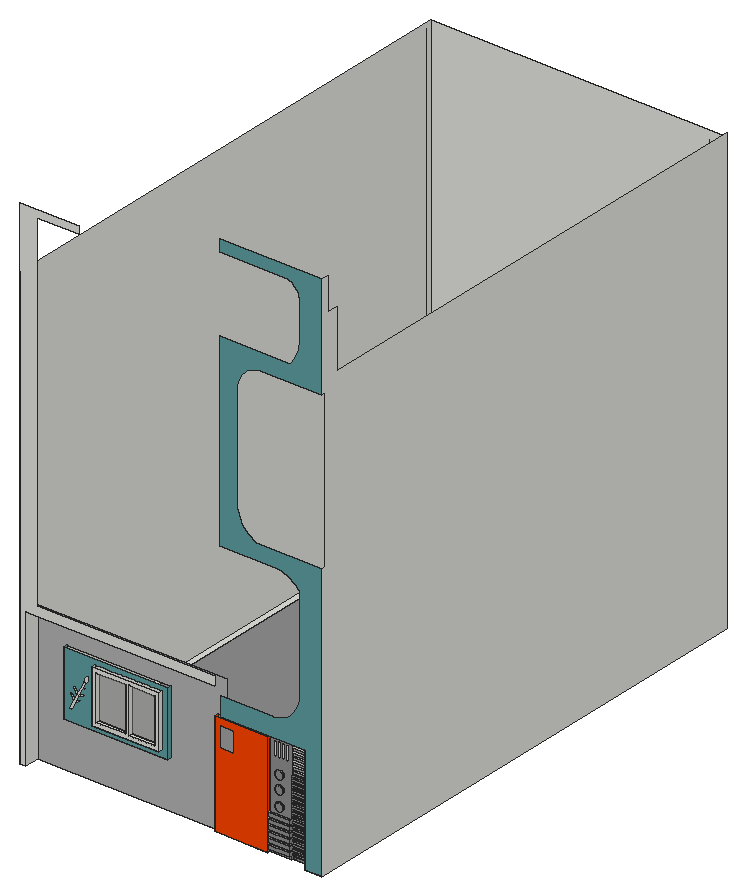
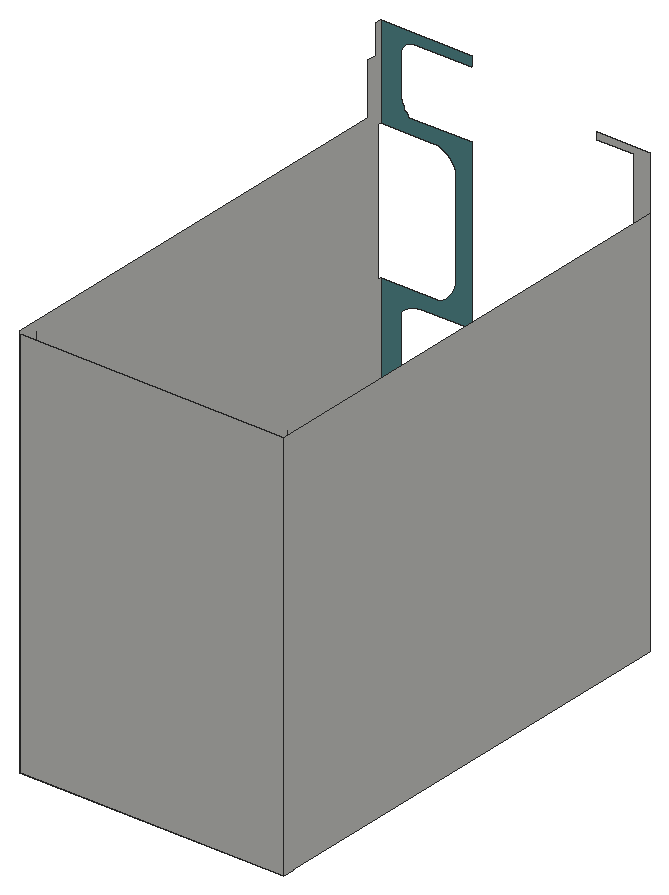
# SketchUp Ruby script. Lengths in inches.
U = 1.inch
M = Sketchup.active_model
def pt(a) = Geom::Point3d.new(a.map { |v| v * U })
def face(e, loops, mat)
  f = e.add_face(loops[0].map { |a| pt(a) })
  loops[1..].each { |l| e.add_face(l.map { |a| pt(a) }).erase! }
  f.material = f.back_material = mat if mat
  f
end
# faces: each face lists its corners as indices into pts; further lists are holes
def faces(e, pts, list, mat = nil) = list.each { |f| face(e, (f[0].is_a?(Array) ? f : [f]).map { |l| l.map { |i| pts[i] } }, mat) }
# xy, xz, yz: faces in a plane at the given z, y or x. An outline is a flat list of corners, or four numbers for a rectangle; further outlines are holes
def ring(l) = l.size == 4 ? [[l[0], l[1]], [l[2], l[1]], [l[2], l[3]], [l[0], l[3]]] : l.each_slice(2).to_a
def flat(e, list, mat, &to3) = list.each { |f| face(e, (f[0].is_a?(Array) ? f : [f]).map { |l| ring(l).map { |u, v| to3.(u, v) } }, mat) }
def xy(e, z, list, mat = nil) = flat(e, list, mat) { |x, y| [x, y, z] }
def xz(e, y, list, mat = nil) = flat(e, list, mat) { |x, z| [x, y, z] }
def yz(e, x, list, mat = nil) = flat(e, list, mat) { |y, z| [x, y, z] }
def lines(e, pts, list) = list.each { |a, b| e.add_line(pt(pts[a]), pt(pts[b])) }
# prism: a flat outline (further loops are holes) pulled along v
def prism(e, loops, v, mat = nil)
  f = face(e, loops, mat); d = Geom::Vector3d.new(v.map { |x| x * U })
  f.pushpull(f.normal.samedirection?(d) ? d.length : -d.length)
end
def box(e, o, s, mat = nil) = prism(e, [[o, [o[0] + s[0], o[1], o[2]], [o[0] + s[0], o[1] + s[1], o[2]], [o[0], o[1] + s[1], o[2]]]], [0, 0, s[2]], mat)
def at(x, y, z, deg = 0) = Geom::Transformation.translation(pt([x, y, z])) * Geom::Transformation.rotation(ORIGIN, Z_AXIS, deg.degrees)
def axes(o, x, y, z) = Geom::Transformation.new([*x, 0, *y, 0, *z, 0, *pt(o).to_a, 1])
def part(name) = M.definitions.add(name)
# library, detail: a bought-in or finely detailed component or shape, given as its bounding box
def library(name, o, s) = part(name).tap { |d| box(d.entities, o, s) }
def detail(e, o, s) = box(e.add_group.entities, o, s)
def put(e, d, t, mat = nil) = e.add_instance(d, t).tap { |i| i.material = mat if mat }
def group(e, t, mat = nil) = e.add_group.tap { |g| g.transformation = t; g.material = mat if mat }.entities
root = M.entities
M.materials.add("Niraj_Hair_Gray").color = [178, 178, 178]
M.materials.add("[0024_OrangeRed]").color = [255, 69, 0]
M.materials.add("[0081_CadetBlue]").color = [95, 158, 160]
M.materials.add("[Color M04]").color = [142, 142, 142]
M.materials.add("[Translucent Glass Gray]").color = [128, 128, 128]
M.materials["[Translucent Glass Gray]"].alpha = 0.5
xy(root,-2,[[198.26,11,216.37,12]])
xy(root,-2,[[230.7,6,230.7,12,198.26,12,198.26,9,153.86,9,153.86,12,5,12,5,414.4375,0,414.4375,0,424.625,245.1875,424.625,245.1875,6]],"[Color M04]")
xy(root,-1.875,[[0,0,5,414.4375]])
xy(root,0.7,[[198.26,9,216.37,11]],"[Color M04]")
xy(root,1.375,[[216.37,11,230.7,12]])
xy(root,2.67,[[216.37,11,230.7,12]],"[Color M04]")
xy(root,3.79,[[198.26,9,216.37,11]],"[Color M04]")
xy(root,4.8125,[[216.37,11,230.7,12]])
xy(root,5.51,[[198.26,9,216.37,11]])
xy(root,6.1,[[216.37,11,230.7,12]])
xy(root,8.25,[[216.37,11,230.7,12]])
xy(root,8.6,[[198.26,9,216.37,11]],"[Color M04]")
xy(root,9.54,[[216.37,11,230.7,12]])
xy(root,10.32,[[198.26,9,216.37,11]])
xy(root,11.6875,[[216.37,11,230.7,12]])
xy(root,12.98,[[216.37,11,230.7,12]])
xy(root,13.42,[[198.26,9,216.37,11]],"[Color M04]")
xy(root,15.125,[[216.37,11,230.7,12]])
xy(root,15.14,[[198.26,9,216.37,11]])
xy(root,16.42,[[216.37,11,230.7,12]])
xy(root,18.23,[[198.26,9,216.37,11]],"[Color M04]")
xy(root,18.5625,[[216.37,11,230.7,12]])
xy(root,19.85,[[216.37,11,230.7,12]])
xy(root,19.95,[[198.26,9,216.37,11]])
xy(root,22,[[216.37,11,230.7,12]])
xy(root,23.04,[[198.26,9,216.37,11]],"[Color M04]")
xy(root,23.29,[[216.37,11,230.7,12]])
xy(root,24.76,[[198.26,9,216.37,11]])
xy(root,25.4375,[[216.37,11,230.7,12]])
xy(root,26.73,[[216.37,11,230.7,12]])
xy(root,27.85,[[198.26,9,216.37,11]],"[Color M04]")
xy(root,28.875,[[216.37,11,230.7,12]])
xy(root,30.17,[[216.37,11,230.7,12]])
xy(root,32.3125,[[216.37,11,230.7,12]])
xy(root,33.6,[[216.37,11,230.7,12]])
xy(root,35.75,[[216.37,11,230.7,12]])
xy(root,37.04,[[216.37,11,230.7,12]])
xy(root,37.67,[[29.19,9,114.82,12]],"[0081_CadetBlue]")
xy(root,39.1875,[[216.37,11,230.7,12]])
xy(root,40.48,[[216.37,11,230.7,12]])
xy(root,42.625,[[216.37,11,230.7,12]])
xy(root,43.17,[[54.96,6,110.28,9]])
xy(root,43.92,[[216.37,11,230.7,12]])
xy(root,46.0625,[[216.37,11,230.7,12]])
xy(root,46.33,[[58.13,6,82.62,9],[85.26,6,107.11,9]])
xy(root,47.35,[[216.37,11,230.7,12]])
xy(root,49.5,[[216.37,11,230.7,12]])
xy(root,50.79,[[216.37,11,230.7,12]])
xy(root,52.9375,[[216.37,11,230.7,12]])
xy(root,54.23,[[216.37,11,230.7,12]])
xy(root,56.375,[[216.37,11,230.7,12]])
xy(root,57.67,[[216.37,11,230.7,12]])
xy(root,59.8125,[[216.37,11,230.7,12]])
xz(root,0,[[0,-1.875,5,-1.875,5,112.3125,161.25,112.3125,161.25,120,14,120,14,407.79,48.4375,407.79,48.4375,414,0,414]])
xz(root,6,[[[54.96,43.17,110.28,86.73],[58.13,46.33,82.62,83.5625],[85.26,46.33,107.11,83.5625]]])
xz(root,6,[[230.7,-2,245.1875,-2,245.1875,226.28,190.26,226.28,188.03,227.37,185.92,228.66,183.95,230.16,182.125,231.84,180.47,233.68,179.01,235.68,177.75,237.82,176.7,240.0625,175.87,242.4,175.28,244.8,174.92,247.25,174.8,249.73,174.8,334.1,174.98,336.86,175.52,339.57,176.41,342.19,177.63,344.68,179.17,346.98,180.99,349.06,183.07,350.88,185.375,352.42,187.86,353.65,190.48,354.54,193.19,355.08,195.95,355.26,245.1875,355.26,245.1875,441.0625,160.53,441.0625,160.53,431.57,212.95,431.57,214.73,431.46,216.48,431.11,218.17,430.54,219.77,429.75,221.25,428.76,222.6,427.58,223.77,426.24,224.76,424.76,225.55,423.16,226.125,421.47,226.47,419.72,226.59,417.9375,226.59,388.52,226.53,386.72,226.36,384.93,226.08,383.15,225.6875,381.39,225.1875,379.66,224.57,377.97,223.86,376.32,223.04,374.72,222.125,373.17,221.11,371.68,220.01,370.26,218.8125,368.91,160.53,368.91,160.53,213.14,206.79,213.14,208.72,213.07,210.64,212.84,212.53,212.45,214.39,211.92,216.19,211.24,217.94,210.42,219.62,209.47,221.22,208.38,222.72,207.17,224.12,205.84,225.42,204.41,226.59,202.88,226.59,125.26,226.39,122.24,225.8,119.26,224.82,116.39,223.48,113.66,221.8,111.14,219.8,108.86,217.51,106.86,214.99,105.17,212.27,103.83,209.4,102.86,206.42,102.26,203.39,102.07,161.25,102.07,161.25,86.5625,230.7,86.5625]],"[0081_CadetBlue]")
xz(root,9,[[[54.96,43.17,110.28,86.73],[58.13,46.33,82.62,83.5625],[85.26,46.33,107.11,83.5625]],[33.9375,47.49,35.62,47.49,38.55,53.26,41.47,59.04,44.14,64.29,46.5,68.96,47.17,70.28,46.5,70.62,45.84,70.96,45.41,70.12,42.7,64.77,40.01,59.47,36.97,53.48],[38.55,53.26,44.04,55.68,43.51,55.74,42.99,55.74,42.46,55.7,41.94,55.61,41.43,55.46,40.9375,55.27,40.47,55.04,40.02,54.76,39.6,54.4375,39.21,54.08,38.86,53.6875],[36.97,53.48,37.22,53.99,37.375,54.53,37.45,55.09,37.43,55.65,37.33,56.2,37.14,56.73,36.87,57.23,36.53,57.67,36.12,58.0625,35.65,58.38,35.15,58.625,34.61,58.78],[41.47,59.04,46.18,60.52,45.76,60.62,45.33,60.68,44.89,60.7,44.46,60.67,44.03,60.6,43.6,60.49,43.2,60.34,42.8,60.15,42.43,59.92,42.08,59.66,41.76,59.36],
  [40.01,59.47,40.1875,59.97,40.29,60.48,40.31,61.01,40.25,61.54,40.12,62.05,39.92,62.54,39.64,62.99,39.3,63.4,38.91,63.75,38.47,64.04,37.99,64.27,37.48,64.42]])
xz(root,9,[[[153.86,-2,198.26,83.875],[157.99,61.11,169.99,78.23]]],"[0024_OrangeRed]")
xz(root,9,[[[29.19,37.67,114.82,90.99],[54.96,43.17,110.28,86.73],[33.9375,47.49,36.97,53.48,36.47,53.68,35.99,53.95,35.56,54.28,35.17,54.67,34.85,55.11,34.59,55.6,34.4,56.11,34.29,56.65,34.26,57.19,34.3,57.74,34.41,58.27,34.61,58.78,35.15,58.625,35.65,58.38,36.12,58.0625,36.53,57.67,36.87,57.23,37.14,56.73,37.33,56.2,37.43,55.65,37.45,55.09,37.375,54.53,37.22,53.99,36.97,53.48,34.61,58.78,34.41,58.27,34.3,57.74,34.26,57.19,34.29,56.65,34.4,56.11,34.59,55.6,34.85,55.11,35.17,54.67,35.56,54.28,35.99,53.95,36.47,53.68,36.97,53.48,40.01,59.47,39.5625,59.69,39.14,59.97,38.76,60.29,38.41,60.65,38.11,61.06,37.86,61.49,37.65,61.95,37.51,62.43,37.41,62.92,37.38,63.42,37.4,63.92,37.48,64.42,37.99,64.27,38.47,64.04,38.91,63.75,39.3,63.4,39.64,62.99,39.92,62.54,40.12,62.05,40.25,61.54,40.31,61.01,40.29,60.48,40.1875,59.97,40.01,59.47,37.48,64.42,37.4,63.92,37.38,63.42,37.41,62.92,37.51,62.43,37.65,61.95,37.86,61.49,38.11,61.06,38.41,60.65,38.76,60.29,39.14,59.97,39.5625,59.69,40.01,59.47,42.7,64.77,42.22,65.04,41.78,65.38,41.4,65.78,41.08,66.23,40.82,66.72,40.65,67.25,40.55,67.79,40.53,68.34,40.6,68.89,40.74,69.43,40.96,69.93,41.26,70.4,41.69,70.09,42.08,69.73,42.42,69.32,42.71,68.87,42.9375,68.38,43.1,67.875,43.2,67.35,43.23,66.82,43.2,66.29,43.1,65.76,42.93,65.26,42.7,64.77,41.26,70.4,40.96,69.93,40.74,69.43,40.6,68.89,40.53,68.34,40.55,67.79,40.65,67.25,40.82,66.72,41.08,66.23,41.4,65.78,41.78,65.38,42.22,65.04,42.7,64.77,45.41,70.12,45.28,70.83,45.25,71.5625,45.33,72.29,45.5,73,45.78,73.67,46.14,74.3,46.6,74.875,47.125,75.38,47.72,75.8,48.37,76.14,49.06,76.38,49.77,76.52,49.9,75.8,49.94,75.07,49.91,74.33,49.81,73.61,49.625,72.9,49.37,72.21,49.04,71.55,48.65,70.93,48.19,70.36,47.68,69.83,47.12,69.36,46.5,68.96,44.14,64.29,44.64,64.2,45.14,64.17,45.65,64.1875,46.15,64.27,46.64,64.41,47.11,64.6,47.55,64.85,47.96,65.14,48.34,65.48,48.68,65.86,48.97,66.27,49.21,66.72,44.14,64.29,44.39,64.73,44.6875,65.13,45.03,65.5,45.41,65.83,45.82,66.12,46.26,66.36,46.73,66.55,47.21,66.7,47.71,66.78,48.21,66.81,48.72,66.79,49.21,66.72,48.97,66.27,48.68,65.86,48.34,65.48,47.96,65.14,47.55,64.85,47.11,64.6,46.64,64.41,46.15,64.27,45.65,64.1875,45.14,64.17,44.64,64.2,44.14,64.29,41.47,59.04,41.9,58.9,42.33,58.8,42.77,58.76,43.22,58.77,43.66,58.83,44.09,58.94,44.51,59.1,44.9,59.3,45.27,59.55,45.61,59.84,45.92,60.16,46.18,60.52,41.47,59.04,41.76,59.36,42.08,59.66,42.43,59.92,42.8,60.15,43.2,60.34,43.6,60.49,44.03,60.6,44.46,60.67,44.89,60.7,45.33,60.68,45.76,60.62,46.18,60.52,45.92,60.16,45.61,59.84,45.27,59.55,44.9,59.3,44.51,59.1,44.09,58.94,43.66,58.83,43.22,58.77,42.77,58.76,42.33,58.8,41.9,58.9,41.47,59.04,38.55,53.26,39.08,53.17,39.61,53.13,40.15,53.15,40.68,53.23,41.19,53.37,41.7,53.56,42.17,53.8,42.625,54.09,43.04,54.43,43.42,54.81,43.75,55.23,44.04,55.68,38.55,53.26,38.86,53.6875,39.21,54.08,39.6,54.4375,40.02,54.76,40.47,55.04,40.9375,55.27,41.43,55.46,41.94,55.61,42.46,55.7,42.99,55.74,43.51,55.74,44.04,55.68,43.75,55.23,43.42,54.81,43.04,54.43,42.625,54.09,42.17,53.8,41.7,53.56,41.19,53.37,40.68,53.23,40.15,53.15,39.61,53.13,39.08,53.17,38.55,53.26,35.62,47.49]]],"[0081_CadetBlue]")
xz(root,9,[[198.26,0.7,216.37,3.79],[198.26,5.51,216.37,8.6],[198.26,10.32,216.37,13.42],[198.26,15.14,216.37,18.23],[198.26,19.95,216.37,23.04],
  [198.26,24.76,216.37,27.85]],"[Color M04]")
xz(root,9,[[58.13,46.33,82.62,83.5625],[85.26,46.33,107.11,83.5625]],"[Translucent Glass Gray]")
xz(root,10,[[206.34,30.52,207.21,30.63,208.03,30.97,208.73,31.5,209.26,32.2,209.6,33.02,209.71,33.89,209.6,34.76,209.26,35.58,208.73,36.28,208.03,36.8125,207.21,37.15,206.34,37.27,205.47,37.15,204.65,36.8125,203.95,36.28,203.42,35.58,203.08,34.76,202.96,33.89,203.08,33.02,203.42,32.2,203.95,31.5,204.65,30.97,205.47,30.63],[206.34,43.2,207.21,43.32,208.03,43.66,208.73,44.19,209.26,44.89,209.6,45.7,209.71,46.58,209.6,47.45,209.26,48.27,208.73,48.96,208.03,49.5,207.21,49.84,206.34,49.95,205.47,49.84,204.65,49.5,203.95,48.96,203.42,48.27,203.08,47.45,202.96,46.58,203.08,45.7,203.42,44.89,203.95,44.19,204.65,43.66,205.47,43.32],[206.34,54.39,207.21,54.51,208.03,54.84,208.73,55.38,209.26,56.08,209.6,56.89,209.71,57.77,209.6,58.64,209.26,59.45,208.73,60.15,208.03,60.6875,207.21,61.03,206.34,61.14,205.47,61.03,204.65,60.6875,203.95,60.15,203.42,59.45,203.08,58.64,202.96,57.77,203.08,56.89,203.42,56.08,203.95,55.38,204.65,54.84,205.47,54.51]],"[Color M04]")
xz(root,11,[[198.26,-2,216.37,0.7],[216.37,1.375,230.7,2.67],[198.26,3.79,216.37,5.51],[216.37,4.8125,230.7,6.1],[216.37,8.25,230.7,9.54],
  [198.26,8.6,216.37,10.32],[216.37,11.6875,230.7,12.98],[198.26,13.42,216.37,15.14],[216.37,15.125,230.7,16.42],[198.26,18.23,216.37,19.95],
  [216.37,18.5625,230.7,19.85],[216.37,22,230.7,23.29],[198.26,23.04,216.37,24.76],[216.37,25.4375,230.7,26.73],[[198.26,27.85,216.37,83.875],[206.34,30.52,205.47,30.63,204.65,30.97,203.95,31.5,203.42,32.2,203.08,33.02,202.96,33.89,203.08,34.76,203.42,35.58,203.95,36.28,204.65,36.8125,205.47,37.15,206.34,37.27,207.21,37.15,208.03,36.8125,208.73,36.28,209.26,35.58,209.6,34.76,209.71,33.89,209.6,33.02,209.26,32.2,208.73,31.5,208.03,30.97,207.21,30.63],[206.34,43.2,205.47,43.32,204.65,43.66,203.95,44.19,203.42,44.89,203.08,45.7,202.96,46.58,203.08,47.45,203.42,48.27,203.95,48.96,204.65,49.5,205.47,49.84,206.34,49.95,207.21,49.84,208.03,49.5,208.73,48.96,209.26,48.27,209.6,47.45,209.71,46.58,209.6,45.7,209.26,44.89,208.73,44.19,208.03,43.66,207.21,43.32],[206.34,54.39,205.47,54.51,204.65,54.84,203.95,55.38,203.42,56.08,203.08,56.89,202.96,57.77,203.08,58.64,203.42,59.45,203.95,60.15,204.65,60.6875,205.47,61.03,206.34,61.14,207.21,61.03,208.03,60.6875,208.73,60.15,209.26,59.45,209.6,58.64,209.71,57.77,209.6,56.89,209.26,56.08,208.73,55.38,208.03,54.84,207.21,54.51],[211.55,69.76,213.55,81.89],[208.18,69.76,210.18,81.89],[204.8,69.76,206.8,81.89],[201.43,69.76,203.43,81.89]],
  [216.37,28.875,230.7,30.17],[216.37,32.3125,230.7,33.6],[216.37,35.75,230.7,37.04],[216.37,39.1875,230.7,40.48],[216.37,42.625,230.7,43.92],
  [216.37,46.0625,230.7,47.35],[216.37,49.5,230.7,50.79],[216.37,52.9375,230.7,54.23],[216.37,56.375,230.7,57.67],[216.37,59.8125,230.7,61.1]],"[Color M04]")
xz(root,12,[[198.26,-2,216.37,-1.9375],[216.37,-2,230.7,-1.9375],[198.26,-1.9375,216.37,-1.875],[198.26,-1.875,216.37,0],[198.26,0,198.26,83.875,216.37,83.875,216.37,81.73,230.7,81.73,230.7,80.4375,216.37,80.4375,216.37,78.29,230.7,78.29,230.7,77,216.37,77,216.37,74.85,230.7,74.85,230.7,73.5625,216.37,73.5625,216.37,71.42,230.7,71.42,230.7,70.125,216.37,70.125,216.37,67.98,230.7,67.98,230.7,66.6875,216.37,66.6875,216.37,64.54,230.7,64.54,230.7,63.25,216.37,63.25,216.37,61.1,230.7,61.1,230.7,59.8125,216.37,59.8125,216.37,57.67,230.7,57.67,230.7,56.375,216.37,56.375,216.37,54.23,230.7,54.23,230.7,52.9375,216.37,52.9375,216.37,50.79,230.7,50.79,230.7,49.5,216.37,49.5,216.37,47.35,230.7,47.35,230.7,46.0625,216.37,46.0625,216.37,43.92,230.7,43.92,230.7,42.625,216.37,42.625,216.37,40.48,230.7,40.48,230.7,39.1875,216.37,39.1875,216.37,37.04,230.7,37.04,230.7,35.75,216.37,35.75,216.37,33.6,230.7,33.6,230.7,32.3125,216.37,32.3125,216.37,30.17,230.7,30.17,230.7,28.875,216.37,28.875,216.37,26.73,230.7,26.73,230.7,25.4375,216.37,25.4375,216.37,23.29,230.7,23.29,230.7,22,216.37,22,216.37,19.85,230.7,19.85,230.7,18.5625,216.37,18.5625,216.37,16.42,230.7,16.42,230.7,15.125,216.37,15.125,216.37,12.98,230.7,12.98,230.7,11.6875,216.37,11.6875,216.37,9.54,230.7,9.54,230.7,8.25,216.37,8.25,216.37,6.1,230.7,6.1,230.7,4.8125,216.37,4.8125,216.37,2.67,230.7,2.67,230.7,1.375,216.37,1.375,216.37,0],
  [29.19,37.67,114.82,81.74]])
xz(root,12,[[[5,-2,153.86,-2,153.86,83.875,230.7,83.875,230.7,86.5625,161.25,86.5625,161.25,112.3125,5,112.3125],[29.19,37.67,114.82,90.99]]],"Niraj_Hair_Gray")
xz(root,12,[[216.37,-1.9375,230.7,0]],"[Color M04]")
xz(root,414.4375,[[0,-2,5,-1.9375],[0,-1.9375,5,-1.875]])
xz(root,424.625,[[0,-2,245.1875,363]])
yz(root,0,[[414.4375,-2,414.4375,-1.875,0,-1.875,0,363,424.625,363,424.625,-2]])
yz(root,5,[[12,-2,414.4375,-1.9375],[12,-1.9375,414.4375,-1.875],[0,-1.875,12,112.3125]])
yz(root,29.19,[[9,37.67,12,90.99]],"[0081_CadetBlue]")
yz(root,54.96,[[6,43.17,9,86.73]])
yz(root,58.13,[[6,46.33,9,83.5625]])
yz(root,82.62,[[6,46.33,9,83.5625]])
yz(root,85.26,[[6,46.33,9,83.5625]])
yz(root,107.11,[[6,46.33,9,83.5625]])
yz(root,110.28,[[6,43.17,9,86.73]])
yz(root,114.82,[[9,37.67,12,90.99]],"[0081_CadetBlue]")
yz(root,153.86,[[9,-2,12,83.875]],"[0024_OrangeRed]")
yz(root,198.26,[[9,-2,11,-1.9375],[11,-2,12,-1.9375],[9,-1.9375,11,-1.875],[11,-1.9375,12,-1.875],[11,-1.875,12,0],
  [11,0,12,0,12,83.875,11,83.875,11,27.85,9,27.85,9,24.76,11,24.76,11,23.04,9,23.04,9,19.95,11,19.95,11,18.23,9,18.23,9,15.14,11,15.14,11,13.42,9,13.42,9,10.32,11,10.32,11,8.6,9,8.6,9,5.51,11,5.51,11,3.79,9,3.79,9,0.7,11,0.7],[9,23.04,11,24.76]])
yz(root,198.26,[[9,27.85,11,83.875]],"[0024_OrangeRed]")
yz(root,198.26,[[9,-1.875,11,0.7],[9,3.79,11,5.51],[9,8.6,11,10.32],[9,13.42,11,15.14],[9,18.23,11,19.95]],"[Color M04]")
yz(root,216.37,[[11,-2,12,-2,12,1.375,11,1.375,11,2.67,12,2.67,12,4.8125,11,4.8125,11,3.79,9,3.79,9,0.7,11,0.7],[9,5.51,11,5.51,11,6.1,12,6.1,12,8.25,11,8.25,11,8.6,9,8.6],[11,9.54,12,9.54,12,11.6875,11,11.6875,11,12.98,12,12.98,12,15.125,11,15.125,11,13.42,9,13.42,9,10.32,11,10.32],[9,15.14,11,15.14,11,16.42,12,16.42,12,18.5625,11,18.5625,11,18.23,9,18.23],[11,19.85,12,19.85,12,22,11,22,11,23.04,9,23.04,9,19.95,11,19.95],
  [11,23.29,12,23.29,12,25.4375,11,25.4375,11,26.73,12,26.73,12,28.875,11,28.875,11,27.85,9,27.85,9,24.76,11,24.76],[11,30.17,12,32.3125],[11,33.6,12,35.75],[11,37.04,12,39.1875],[11,40.48,12,42.625],
  [11,43.92,12,46.0625],[11,47.35,12,49.5],[11,50.79,12,52.9375],[11,54.23,12,56.375],[11,57.67,12,59.8125]],"[Color M04]")
yz(root,230.7,[[6,-2,12,-1.9375],[6,-1.9375,12,-1.875],[11,1.375,12,2.67],[11,4.8125,12,6.1],[11,8.25,12,9.54],
  [11,11.6875,12,12.98],[11,15.125,12,16.42],[11,18.5625,12,19.85],[11,22,12,23.29],[11,25.4375,12,26.73],
  [11,28.875,12,30.17],[11,32.3125,12,33.6],[11,35.75,12,37.04],[11,39.1875,12,40.48],[11,42.625,12,43.92],
  [11,46.0625,12,47.35],[11,49.5,12,50.79],[11,52.9375,12,54.23],[11,56.375,12,57.67],[11,59.8125,12,61.1]])
yz(root,230.7,[[6,-1.875,6,86.5625,12,86.5625,12,81.73,11,81.73,11,80.4375,12,80.4375,12,78.29,11,78.29,11,77,12,77,12,74.85,11,74.85,11,73.5625,12,73.5625,12,71.42,11,71.42,11,70.125,12,70.125,12,67.98,11,67.98,11,66.6875,12,66.6875,12,64.54,11,64.54,11,63.25,12,63.25,12,61.1,11,61.1,11,59.8125,12,59.8125,12,57.67,11,57.67,11,56.375,12,56.375,12,54.23,11,54.23,11,52.9375,12,52.9375,12,50.79,11,50.79,11,49.5,12,49.5,12,47.35,11,47.35,11,46.0625,12,46.0625,12,43.92,11,43.92,11,42.625,12,42.625,12,40.48,11,40.48,11,39.1875,12,39.1875,12,37.04,11,37.04,11,35.75,12,35.75,12,33.6,11,33.6,11,32.3125,12,32.3125,12,30.17,11,30.17,11,28.875,12,28.875,12,26.73,11,26.73,11,25.4375,12,25.4375,12,23.29,11,23.29,11,22,12,22,12,19.85,11,19.85,11,18.5625,12,18.5625,12,16.42,11,16.42,11,15.125,12,15.125,12,12.98,11,12.98,11,11.6875,12,11.6875,12,9.54,11,9.54,11,8.25,12,8.25,12,6.1,11,6.1,11,4.8125,12,4.8125,12,2.67,11,2.67,11,1.375,12,1.375,12,-1.875]],"[0081_CadetBlue]")
yz(root,245.1875,[[6,-2,424.625,-2,424.625,366,21,366,21,414,12,414,12,441.0625,6,441.0625,6,355.26,9,355.26,9,297.89,9.125,297.89,9.125,293.27,9,293.27,9,226.28,6,226.28]])
p = [[205.47,11,30.63],[206.34,11,30.52],[206.34,10,30.52],[205.47,10,30.63],[207.21,11,30.63],[207.21,10,30.63],
  [204.65,11,30.97],[204.65,10,30.97],[208.03,11,30.97],[208.03,10,30.97],[203.95,11,31.5],[203.95,10,31.5],
  [208.73,11,31.5],[208.73,10,31.5],[203.42,11,32.2],[203.42,10,32.2],[209.26,11,32.2],[209.26,10,32.2],
  [203.08,11,33.02],[203.08,10,33.02],[209.6,11,33.02],[209.6,10,33.02],[202.96,11,33.89],[202.96,10,33.89],
  [209.71,11,33.89],[209.71,10,33.89],[203.08,11,34.76],[203.08,10,34.76],[209.6,11,34.76],[209.6,10,34.76],
  [203.42,11,35.58],[203.42,10,35.58],[209.26,11,35.58],[209.26,10,35.58],[203.95,11,36.28],[203.95,10,36.28],
  [208.73,11,36.28],[208.73,10,36.28],[204.65,11,36.8125],[204.65,10,36.8125],[208.03,11,36.8125],[208.03,10,36.8125],
  [205.47,11,37.15],[205.47,10,37.15],[207.21,11,37.15],[207.21,10,37.15],[206.34,11,37.27],[206.34,10,37.27],
  [205.47,11,43.32],[206.34,11,43.2],[206.34,10,43.2],[205.47,10,43.32],[207.21,11,43.32],[207.21,10,43.32],
  [204.65,11,43.66],[204.65,10,43.66],[208.03,11,43.66],[208.03,10,43.66],[203.95,11,44.19],[203.95,10,44.19],
  [208.73,11,44.19],[208.73,10,44.19],[203.42,11,44.89],[203.42,10,44.89],[209.26,11,44.89],[209.26,10,44.89],
  [203.08,11,45.7],[203.08,10,45.7],[209.6,11,45.7],[209.6,10,45.7],[202.96,11,46.58],[202.96,10,46.58],
  [209.71,11,46.58],[209.71,10,46.58],[203.08,11,47.45],[203.08,10,47.45],[209.6,11,47.45],[209.6,10,47.45],
  [203.42,11,48.27],[203.42,10,48.27],[209.26,11,48.27],[209.26,10,48.27],[203.95,11,48.96],[203.95,10,48.96],
  [208.73,11,48.96],[208.73,10,48.96],[204.65,11,49.5],[204.65,10,49.5],[208.03,11,49.5],[208.03,10,49.5],
  [205.47,11,49.84],[205.47,10,49.84],[207.21,11,49.84],[207.21,10,49.84],[206.34,11,49.95],[206.34,10,49.95],
  [205.47,11,54.51],[206.34,11,54.39],[206.34,10,54.39],[205.47,10,54.51],[207.21,11,54.51],[207.21,10,54.51],
  [204.65,11,54.84],[204.65,10,54.84],[208.03,11,54.84],[208.03,10,54.84],[203.95,11,55.38],[203.95,10,55.38],
  [208.73,11,55.38],[208.73,10,55.38],[203.42,11,56.08],[203.42,10,56.08],[209.26,11,56.08],[209.26,10,56.08],
  [203.08,11,56.89],[203.08,10,56.89],[209.6,11,56.89],[209.6,10,56.89],[202.96,11,57.77],[202.96,10,57.77],
  [209.71,11,57.77],[209.71,10,57.77],[203.08,11,58.64],[203.08,10,58.64],[209.6,11,58.64],[209.6,10,58.64],
  [203.42,11,59.45],[203.42,10,59.45],[209.26,11,59.45],[209.26,10,59.45],[203.95,11,60.15],[203.95,10,60.15],
  [208.73,11,60.15],[208.73,10,60.15],[204.65,11,60.6875],[204.65,10,60.6875],[208.03,11,60.6875],[208.03,10,60.6875],
  [5,414.4375,-1.875],[5,414.4375,363],[241.9375,414.4375,-2],[241.9375,414.4375,-1.9375],[238.75,414.4375,-2],[238.75,414.4375,363],
  [241.9375,6,-1.9375],[241.9375,6,-2]]
faces(root,p,[[0,1,2,3],[1,4,5,2],[6,0,3,7],[4,8,9,5],[10,6,7,11],[8,12,13,9],[14,10,11,15],[12,16,17,13],
  [18,14,15,19],[16,20,21,17],[22,18,19,23],[20,24,25,21],[26,22,23,27],[24,28,29,25],[30,26,27,31],[28,32,33,29],
  [34,30,31,35],[32,36,37,33],[38,34,35,39],[36,40,41,37],[42,38,39,43],[40,44,45,41],[46,42,43,47],[44,46,47,45],
  [48,49,50,51],[49,52,53,50],[54,48,51,55],[52,56,57,53],[58,54,55,59],[56,60,61,57],[62,58,59,63],[60,64,65,61],
  [66,62,63,67],[64,68,69,65],[70,66,67,71],[68,72,73,69],[74,70,71,75],[72,76,77,73],[78,74,75,79],[76,80,81,77],
  [82,78,79,83],[80,84,85,81],[86,82,83,87],[84,88,89,85],[90,86,87,91],[88,92,93,89],[94,90,91,95],[92,94,95,93],
  [96,97,98,99],[97,100,101,98],[102,96,99,103],[100,104,105,101],[106,102,103,107],[104,108,109,105],[110,106,107,111],[108,112,113,109],
  [114,110,111,115],[112,116,117,113],[118,114,115,119],[116,120,121,117],[122,118,119,123],[120,124,125,121],[126,122,123,127],[124,128,129,125],
  [130,126,127,131],[128,132,133,129],[134,130,131,135],[132,136,137,133]],"[Color M04]")
lines(root,p,[[138,139],[140,141],[142,143],[144,145]])
